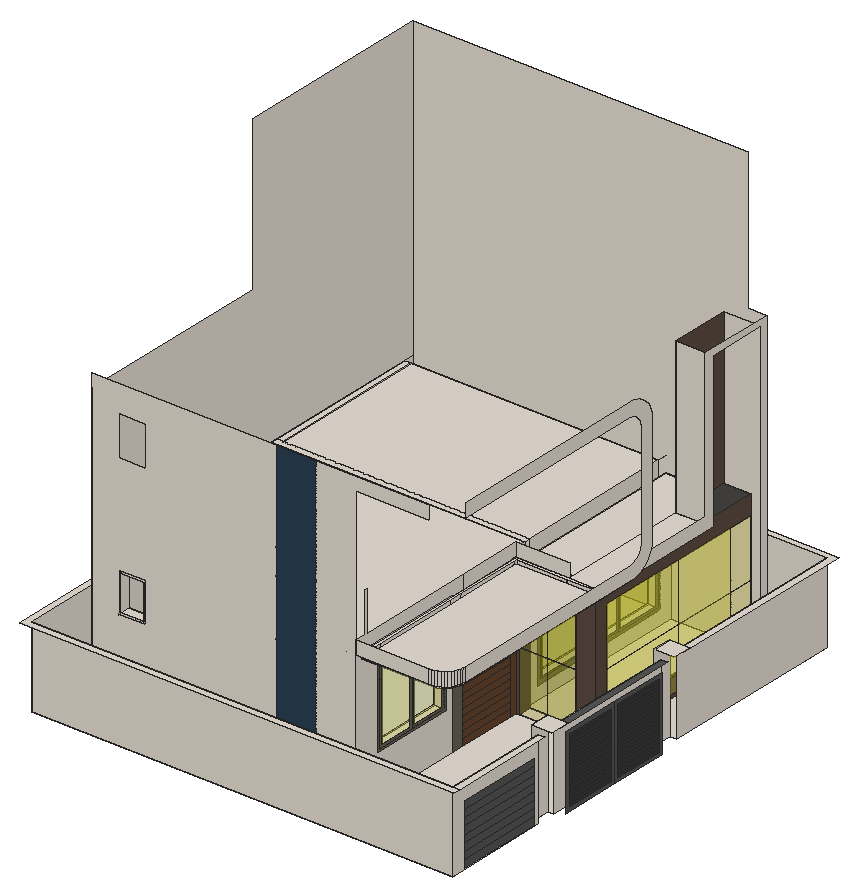
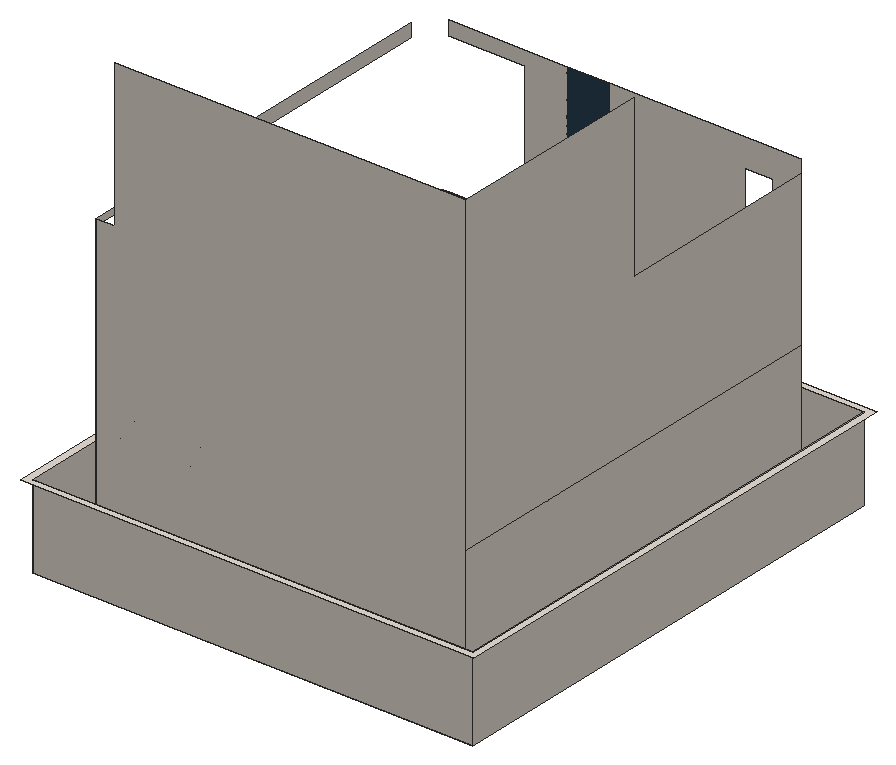
# SketchUp Ruby script. Lengths in inches.
U = 1.inch
M = Sketchup.active_model
def pt(a) = Geom::Point3d.new(a.map { |v| v * U })
def face(e, loops, mat)
  f = e.add_face(loops[0].map { |a| pt(a) })
  loops[1..].each { |l| e.add_face(l.map { |a| pt(a) }).erase! }
  f.material = f.back_material = mat if mat
  f
end
# faces: each face lists its corners as indices into pts; further lists are holes
def faces(e, pts, list, mat = nil) = list.each { |f| face(e, (f[0].is_a?(Array) ? f : [f]).map { |l| l.map { |i| pts[i] } }, mat) }
# xy, xz, yz: faces in a plane at the given z, y or x. An outline is a flat list of corners, or four numbers for a rectangle; further outlines are holes
def ring(l) = l.size == 4 ? [[l[0], l[1]], [l[2], l[1]], [l[2], l[3]], [l[0], l[3]]] : l.each_slice(2).to_a
def flat(e, list, mat, &to3) = list.each { |f| face(e, (f[0].is_a?(Array) ? f : [f]).map { |l| ring(l).map { |u, v| to3.(u, v) } }, mat) }
def xy(e, z, list, mat = nil) = flat(e, list, mat) { |x, y| [x, y, z] }
def xz(e, y, list, mat = nil) = flat(e, list, mat) { |x, z| [x, y, z] }
def yz(e, x, list, mat = nil) = flat(e, list, mat) { |y, z| [x, y, z] }
def lines(e, pts, list) = list.each { |a, b| e.add_line(pt(pts[a]), pt(pts[b])) }
# prism: a flat outline (further loops are holes) pulled along v
def prism(e, loops, v, mat = nil)
  f = face(e, loops, mat); d = Geom::Vector3d.new(v.map { |x| x * U })
  f.pushpull(f.normal.samedirection?(d) ? d.length : -d.length)
end
def box(e, o, s, mat = nil) = prism(e, [[o, [o[0] + s[0], o[1], o[2]], [o[0] + s[0], o[1] + s[1], o[2]], [o[0], o[1] + s[1], o[2]]]], [0, 0, s[2]], mat)
def at(x, y, z, deg = 0) = Geom::Transformation.translation(pt([x, y, z])) * Geom::Transformation.rotation(ORIGIN, Z_AXIS, deg.degrees)
def axes(o, x, y, z) = Geom::Transformation.new([*x, 0, *y, 0, *z, 0, *pt(o).to_a, 1])
def part(name) = M.definitions.add(name)
# library, detail: a bought-in or finely detailed component or shape, given as its bounding box
def library(name, o, s) = part(name).tap { |d| box(d.entities, o, s) }
def detail(e, o, s) = box(e.add_group.entities, o, s)
def put(e, d, t, mat = nil) = e.add_instance(d, t).tap { |i| i.material = mat if mat }
def group(e, t, mat = nil) = e.add_group.tap { |g| g.transformation = t; g.material = mat if mat }.entities
root = M.entities
M.materials.add("Carpet_04_1K").color = [43, 65, 85]
M.materials.add("Glass_Basic_01").color = [255, 251, 32]
M.materials["Glass_Basic_01"].alpha = 0.25
M.materials.add("Glass_Basic_1").color = [186, 185, 19]
M.materials["Glass_Basic_1"].alpha = 0.25
M.materials.add("Glass_Safety_01").color = [204, 235, 244]
M.materials["Glass_Safety_01"].alpha = 0.25
M.materials.add("M06_Steel_Smoke").color = [86, 86, 86]
M.materials.add("M07_Charcoal_Gleam").color = [58, 58, 58]
M.materials.add("Marble_01_1K").color = [230, 221, 211]
M.materials.add("Plaster_04_1K").color = [106, 98, 87]
M.materials.add("Wood_Floor_12_1K").color = [92, 75, 65]
M.materials.add("Wood_Planks_01_1K").color = [69, 67, 63]
M.materials.add("Wood_Veneer_15_1K").color = [103, 69, 45]
xy(root,-6,[[[6,6,384,6,384,102,378,102,378,120,384,120,384,240,378,240,378,258,384,258,384,426,6,426],[36,36,36,396,354,396,354,390,345,390,345,216,273,216,273,36]],[36,36,201,396],[201,36,237,396],[237,36,273,36,273,216,276,216,276,228,273,228,273,390,354,390,354,396,237,396],[276,216,327,228],
  [327,216,345,228],[273,228,327,390],[327,228,345,390]],"Marble_01_1K")
xy(root,-3,[[327,228,333,228,327,390],[333,228,345,228,345,390,327,390]],"Wood_Floor_12_1K")
xy(root,0,[[42,45,264,237],[42,243,264,387]],"Marble_01_1K")
xy(root,9,[[264,243,273,375]],"Marble_01_1K")
xy(root,33,[[264,63,273,135]],"Marble_01_1K")
xy(root,66,[[384,120,390,240]],"M06_Steel_Smoke")
xy(root,66,[[0,0,390,0,390,6,6,6,6,426,384,426,384,258,390,258,390,432,0,432],[384,6,390,102]],"Marble_01_1K")
xy(root,72,[[378,102,396,120],[378,240,396,258]],"Marble_01_1K")
xy(root,80,[[62,36,82,45]],"Marble_01_1K")
xy(root,99,[[264,243,273,375]],"Marble_01_1K")
xy(root,102,[[333,228,327.22,384,333,384]],"Marble_01_1K")
xy(root,102,[[276,216,327,228],[333,228,333,384,327.22,384,327,390,345,390,345,228],[273,384,273,390,327,390,327.22,384]],"Wood_Floor_12_1K")
xy(root,111,[[264,63,273,135]],"Marble_01_1K")
xy(root,112,[[62,36,82,45]],"Marble_01_1K")
xy(root,114,[[273,228,333,384]],"Marble_01_1K")
xy(root,117,[[276,39,276,213,354,213,354,53.96,353.89,52,353.53,50.07,352.91,48.21,352.05,46.44,350.96,44.81,349.67,43.33,348.19,42.04,346.56,40.95,344.79,40.09,342.93,39.47,341,39.11,339.04,39]],"Marble_01_1K")
xy(root,120,[[[273,36,273,216,357,216,357,54,356.87,51.64,356.43,49.32,355.6875,47.08,354.66,44.95,353.35,42.98,351.79,41.21,350.02,39.65,348.05,38.34,345.92,37.3125,343.68,36.57,341.36,36.13,339,36],[276,39,339.04,39,341,39.11,342.93,39.47,344.79,40.09,346.56,40.95,348.19,42.04,349.67,43.33,350.96,44.81,352.05,46.44,352.91,48.21,353.53,50.07,353.89,52,354,53.96,354,213,276,213]],[36,45,42,237],[42,45,264,237],[321,216,345,336],[345,216,345,336,354,336,354,240,357,240,357,216],
  [36,237,264,243],[354,240,357,240.76],[36,243,42,387],[42,243,264,387]],"Marble_01_1K")
xy(root,120,[[321,336,345,390]],"Wood_Planks_01_1K")
xz(root,6,[[6,-6,384,66]],"Marble_01_1K")
xz(root,36,[[201,-6,237,264]],"Carpet_04_1K")
xz(root,36,[[[36,-6,201,264],[60,204,84,240],[60,78,84,114]],[237,-6,273,-6,273,252,339,252,339,264,237,264],[[60,78,84,114],[62,80,82,112]],[273,120,339,132]],"Marble_01_1K")
xz(root,39,[[276,117,339.04,120]],"Marble_01_1K")
xz(root,45,[[[42,0,264,120],[62,80,82,112]]],"Marble_01_1K")
xz(root,63,[[264,33,273,111]],"Marble_01_1K")
xz(root,135,[[264,33,273,111]],"Marble_01_1K")
xz(root,213,[[276,117,321,120],[321,117,345,120],[345,117,354,120]],"Marble_01_1K")
xz(root,216,[[276,-6,301.5,48],[301.5,-6,327,48],[276,48,301.5,102],[301.5,48,327,102]],"Glass_Basic_1")
xz(root,216,[[273,120,321,132]],"Marble_01_1K")
xz(root,216,[[273,-6,276,-6,276,102,327,102,327,-6,345,-6,345,120,273,120]],"Wood_Floor_12_1K")
xz(root,228,[[276,-6,327,102]],"Glass_Basic_1")
xz(root,228,[[273,-6,273,114,333,114,333,108,327,108,327,102,276,102,276,-6],[327,-3,333,108],[333,-3,345,102]],"Wood_Floor_12_1K")
xz(root,237,[[42,0,264,120]],"Marble_01_1K")
xz(root,243,[[42,0,264,120],[264,9,273,99]],"Marble_01_1K")
xz(root,336,[[321,120,354,258]],"Marble_01_1K")
xz(root,375,[[264,9,273,99]],"Marble_01_1K")
xz(root,384,[[273,102,333,114]],"Wood_Floor_12_1K")
xz(root,387,[[42,0,264,120]],"Marble_01_1K")
xz(root,390,[[273,-6,327,102],[345,-6,354,-6,354,258,321,258,321,120,345,120],[327,-3,345,102],[333,102,345,120]],"Marble_01_1K")
xz(root,396,[[36,-6,36,390,337.5,390,337.5,264,354,264,354,-6]],"Marble_01_1K")
xz(root,426,[[6,-6,384,66]],"Marble_01_1K")
yz(root,6,[[6,-6,426,66]],"Marble_01_1K")
yz(root,36,[[36,-6,396,120],[36,120,36,252,216,252,216,390,396,390,396,120]],"Marble_01_1K")
yz(root,42,[[45,0,237,120],[243,0,387,120]],"Marble_01_1K")
yz(root,62,[[36,80,45,112]],"Marble_01_1K")
yz(root,82,[[36,80,45,112]],"Marble_01_1K")
yz(root,264,[[243,9,375,99]],"Glass_Basic_1")
yz(root,264,[[63,33,135,111]],"Glass_Safety_01")
yz(root,264,[[[45,0,237,120],[63,33,135,111]],[243,0,243,9,375,9,375,99,243,99,243,120,387,120,387,0]],"Marble_01_1K")
yz(root,273,[[65,35,97,109],[101,35,133,109]],"Glass_Basic_01")
yz(root,273,[[245,11,285,97],[289,11,329,97],[333,11,373,97]],"Glass_Basic_1")
yz(root,273,[[[36,-6,144,120],[60,30,138,114]],[[228,-6,390,-6,390,102,384,102,384,114,228,114],[240,6,378,102]],[36,120,156,120,156,132,48,132,48,168,46,168,46,132,36,132],[156,120,216,132]],"Marble_01_1K")
yz(root,273,[[144,-6,156,120],[[240,6,378,102],[243,9,375,99]],[[243,9,287,99],[245,11,285,97]],[[287,9,331,99],[289,11,329,97]],[[331,9,375,99],[333,11,373,97]],
  [[60,30,138,114],[63,33,135,111]],[[63,33,99,111],[65,35,97,109]],[[99,33,135,111],[101,35,133,109]]],"Plaster_04_1K")
yz(root,273,[[156,-6,210,0.05],[210,-6,216,120],[156,0.05,210,6.1],[156,6.1,210,12.15],[156,12.15,210,18.21],
  [156,18.21,210,24.26],[156,24.26,210,30.31],[156,30.31,210,36.36],[156,36.36,210,42.41],[156,42.41,210,48.46],
  [156,48.46,210,54.51],[156,54.51,210,60.5625],[156,60.5625,210,66.62],[156,66.62,210,72.67],[156,72.67,210,78.72],
  [156,78.72,210,84.77],[156,84.77,210,90.82],[156,90.82,210,96.87],[156,96.87,210,102.92],[156,102.92,210,108.97],
  [156,108.97,210,115.03],[156,115.03,210,120]],"Wood_Veneer_15_1K")
yz(root,276,[[39,117,60,120],[60,117,138,120],[138,117,150,120],[150,117,210,120],[210,117,213,120]],"Marble_01_1K")
yz(root,276,[[216,-6,228,102]],"Wood_Floor_12_1K")
yz(root,321,[[336,120,390,258]],"Wood_Floor_12_1K")
yz(root,327,[[216,-6,228,102]],"Marble_01_1K")
yz(root,327,[[228,-6,390,-3]],"Wood_Floor_12_1K")
yz(root,333,[[228,102,384,114]],"Marble_01_1K")
yz(root,345,[[228,-3,309,49.5],[309,-3,390,49.5],[228,49.5,309,102],[309,49.5,390,102]],"Glass_Basic_01")
yz(root,345,[[216,-6,390,-6,390,-3,228,-3,228,102,390,102,390,120,216,120]],"Wood_Floor_12_1K")
yz(root,354,[[390,-6,396,-6,396,264,327,264,327,132,260.89,132,260.73,131.73,260.34,131.08,259.93,130.45,259.49,129.83,259.04,129.22,258.57,128.63,258.08,128.06,257.57,127.5,257.04,126.96,256.5,126.43,255.94,125.92,255.37,125.43,254.78,124.96,254.17,124.51,253.55,124.07,252.92,123.66,252.27,123.27,251.61,122.89,250.94,122.54,250.26,122.21,249.57,121.91,248.87,121.62,248.16,121.36,247.45,121.12,246.72,120.9,245.99,120.7,245.26,120.53,244.51,120.38,243.77,120.26,243.02,120.16,242.27,120.08,241.51,120.03,240.76,120,240,120,336,120,336,258,390,258],[53.96,117,213,120]],"Marble_01_1K")
yz(root,357,[[54,120,240.76,120,241.51,120.03,242.27,120.08,243.02,120.16,243.77,120.26,244.51,120.38,245.26,120.53,245.99,120.7,246.72,120.9,247.45,121.12,248.16,121.36,248.87,121.62,249.57,121.91,250.26,122.21,250.94,122.54,251.61,122.89,252.27,123.27,252.92,123.66,253.55,124.07,254.17,124.51,254.78,124.96,255.37,125.43,255.94,125.92,256.5,126.43,257.04,126.96,257.57,127.5,258.08,128.06,258.57,128.63,259.04,129.22,259.49,129.83,259.93,130.45,260.34,131.08,260.73,131.73,260.89,132,261.11,132.39,261.46,133.06,261.79,133.74,262.09,134.43,262.38,135.13,262.64,135.84,262.88,136.55,263.1,137.28,263.3,138.01,263.47,138.74,263.62,139.49,263.74,140.23,263.84,140.98,263.92,141.73,263.97,142.49,264,143.24,264,240,263.97,240.75,263.91,241.49,263.84,242.24,263.74,242.98,263.62,243.72,263.47,244.45,263.31,245.18,263.12,245.91,262.91,246.625,262.68,247.34,262.42,248.04,262.15,248.74,261.85,249.43,261.54,250.11,261.2,250.77,260.84,251.43,260.46,252.08,260.07,252.71,259.65,253.34,259.22,253.95,258.77,254.54,258.3,255.125,257.81,255.69,257.3,256.25,256.78,256.78,256.25,257.3,255.69,257.81,255.125,258.3,254.54,258.77,253.95,259.22,253.34,259.65,252.71,260.07,252.08,260.46,251.43,260.84,250.77,261.2,250.11,261.54,249.43,261.85,248.74,262.15,248.04,262.42,247.34,262.68,246.625,262.91,245.91,263.12,245.18,263.31,244.45,263.47,243.72,263.62,242.98,263.74,242.24,263.84,241.49,263.91,240.75,263.97,240,264,54,264,54,252,240,252,240.36,251.95,240.72,251.89,241.08,251.82,241.44,251.74,241.79,251.65,242.14,251.55,242.49,251.4375,242.83,251.32,243.18,251.2,243.52,251.06,243.85,250.92,244.51,250.6,244.83,250.43,245.47,250.07,245.77,249.875,246.08,249.67,246.375,249.46,246.67,249.24,246.95,249.02,247.24,248.78,247.51,248.54,247.78,248.29,248.04,248.04,248.29,247.78,248.54,247.51,248.78,247.24,249.02,246.95,249.24,246.67,249.46,246.375,249.67,246.08,249.875,245.77,250.07,245.47,250.43,244.83,250.6,244.51,250.92,243.85,251.06,243.52,251.2,243.18,251.32,242.83,251.4375,242.49,251.55,242.14,251.65,241.79,251.74,241.44,251.82,241.08,251.89,240.72,251.95,240.36,252,240,252,144,251.98,143.63,251.9,142.89,251.84,142.52,251.77,142.15,251.7,141.79,251.61,141.43,251.51,141.07,251.4,140.71,251.28,140.36,251.15,140.01,251.01,139.67,250.86,139.33,250.7,138.99,250.53,138.66,250.35,138.34,250.16,138.02,249.96,137.7,249.75,137.39,249.53,137.09,249.31,136.8,248.83,136.22,248.58,135.95,248.32,135.68,248.05,135.42,247.78,135.17,247.2,134.69,246.91,134.47,246.61,134.25,246.3,134.04,245.98,133.84,245.66,133.65,245.34,133.47,245.01,133.3,244.67,133.14,244.33,132.99,243.99,132.85,243.64,132.72,243.29,132.6,242.93,132.49,242.57,132.39,242.21,132.3,241.85,132.23,241.48,132.16,241.11,132.1,240.37,132.02,240,132,54,132]],"Marble_01_1K")
yz(root,378,[[102,-6,120,72],[240,-6,258,72]],"Marble_01_1K")
yz(root,384,[[6,-6,102,66],[120,-6,240,66],[258,-6,426,66]],"Marble_01_1K")
yz(root,390,[[[126,-6,180,60],[129,-3,177,57]],[[180,-6,234,60],[183,-3,231,57]],[12,0,90,6.75],[12,6.75,90,13.5],[12,13.5,90,20.25],
  [12,20.25,90,27],[12,27,90,33.75],[12,33.75,90,40.5],[12,40.5,90,47.25],[12,47.25,90,54]],"M06_Steel_Smoke")
yz(root,390,[[129,-3,177,0],[183,-3,231,0],[129,0,177,3],[183,0,231,3],[129,3,177,6],
  [183,3,231,6],[129,6,177,9],[183,6,231,9],[129,9,177,12],[183,9,231,12],
  [129,12,177,15],[183,12,231,15],[129,15,177,18],[183,15,231,18],[129,18,177,21],
  [183,18,231,21],[129,21,177,24],[183,21,231,24],[129,24,177,27],[183,24,231,27],
  [129,27,177,30],[183,27,231,30],[129,30,177,33],[183,30,231,33],[129,33,177,36],
  [183,33,231,36],[129,36,177,39],[183,36,231,39],[129,39,177,42],[183,39,231,42],
  [129,42,177,45],[183,42,231,45],[129,45,177,48],[183,45,231,48],[129,48,177,51],
  [183,48,231,51],[129,51,177,54],[183,51,231,54],[129,54,177,57],[183,54,231,57]],"M07_Charcoal_Gleam")
p = [[327.22,384,102],[333,228,102],[333,228,-3],[327,390,-3],[327,390,102],[341,39.11,120],
  [339.04,39,120],[339.04,39,117],[341,39.11,117],[342.93,39.47,120],[342.93,39.47,117],[344.79,40.09,120],
  [344.79,40.09,117],[346.56,40.95,120],[346.56,40.95,117],[348.19,42.04,120],[348.19,42.04,117],[349.67,43.33,120],
  [349.67,43.33,117],[350.96,44.81,120],[350.96,44.81,117],[352.05,46.44,120],[352.05,46.44,117],[352.91,48.21,120],
  [352.91,48.21,117],[353.53,50.07,120],[353.53,50.07,117],[353.89,52,120],[353.89,52,117],[354,53.96,120],
  [354,53.96,117],[341.36,36.13,132],[339,36,132],[339,36,120],[341.36,36.13,120],[343.68,36.57,132],
  [343.68,36.57,120],[345.92,37.3125,132],[345.92,37.3125,120],[348.05,38.34,132],[348.05,38.34,120],[350.02,39.65,132],
  [350.02,39.65,120],[351.79,41.21,132],[351.79,41.21,120],[353.35,42.98,132],[353.35,42.98,120],[354.66,44.95,132],
  [354.66,44.95,120],[355.6875,47.08,132],[355.6875,47.08,120],[356.43,49.32,132],[356.43,49.32,120],[356.87,51.64,132],
  [356.87,51.64,120],[357,54,132],[357,54,120],[357,241.51,120.03],[357,240.76,120],[354,240.76,120],
  [354,241.51,120.03],[357,242.27,120.08],[354,242.27,120.08],[357,243.02,120.16],[354,243.02,120.16],[357,243.77,120.26],
  [354,243.77,120.26],[357,244.51,120.38],[354,244.51,120.38],[357,245.26,120.53],[354,245.26,120.53],[357,245.99,120.7],
  [354,245.99,120.7],[357,246.72,120.9],[354,246.72,120.9],[357,247.45,121.12],[354,247.45,121.12],[357,248.16,121.36],
  [354,248.16,121.36],[357,248.87,121.62],[354,248.87,121.62],[357,249.57,121.91],[354,249.57,121.91],[357,250.26,122.21],
  [354,250.26,122.21],[357,250.94,122.54],[354,250.94,122.54],[357,251.61,122.89],[354,251.61,122.89],[357,252.27,123.27],
  [354,252.27,123.27],[357,252.92,123.66],[354,252.92,123.66],[357,253.55,124.07],[354,253.55,124.07],[357,254.17,124.51],
  [354,254.17,124.51],[357,254.78,124.96],[354,254.78,124.96],[357,255.37,125.43],[354,255.37,125.43],[357,255.94,125.92],
  [354,255.94,125.92],[357,256.5,126.43],[354,256.5,126.43],[357,257.04,126.96],[354,257.04,126.96],[357,257.57,127.5],
  [354,257.57,127.5],[357,258.08,128.06],[354,258.08,128.06],[357,258.57,128.63],[354,258.57,128.63],[357,259.04,129.22],
  [354,259.04,129.22],[357,259.49,129.83],[354,259.49,129.83],[357,259.93,130.45],[354,259.93,130.45],[357,260.34,131.08],
  [354,260.34,131.08],[357,260.73,131.73],[354,260.73,131.73],[321,396,120],[321,390,120],[273,396,102],
  [273,390,102],[333,390,102],[333,396,102],[264,387,120],[264,396,120],[264,45,120],
  [264,36,120]]
faces(root,p,[[0,1,2,3,4]],"Glass_Basic_01")
faces(root,p,[[5,6,7,8],[9,5,8,10],[11,9,10,12],[13,11,12,14],[15,13,14,16],[17,15,16,18],[19,17,18,20],[21,19,20,22],
  [23,21,22,24],[25,23,24,26],[27,25,26,28],[29,27,28,30],[31,32,33,34],[35,31,34,36],[37,35,36,38],[39,37,38,40],
  [41,39,40,42],[43,41,42,44],[45,43,44,46],[47,45,46,48],[49,47,48,50],[51,49,50,52],[53,51,52,54],[55,53,54,56],
  [57,58,59,60],[61,57,60,62],[63,61,62,64],[65,63,64,66],[67,65,66,68],[69,67,68,70],[71,69,70,72],[73,71,72,74],
  [75,73,74,76],[77,75,76,78],[79,77,78,80],[81,79,80,82],[83,81,82,84],[85,83,84,86],[87,85,86,88],[89,87,88,90],
  [91,89,90,92],[93,91,92,94],[95,93,94,96],[97,95,96,98],[99,97,98,100],[101,99,100,102],[103,101,102,104],[105,103,104,106],
  [107,105,106,108],[109,107,108,110],[111,109,110,112],[113,111,112,114],[115,113,114,116],[117,115,116,118],[119,117,118,120],[121,119,120,122]],"Marble_01_1K")
lines(root,p,[[123,124],[125,126],[127,128],[129,130],[131,132]])
